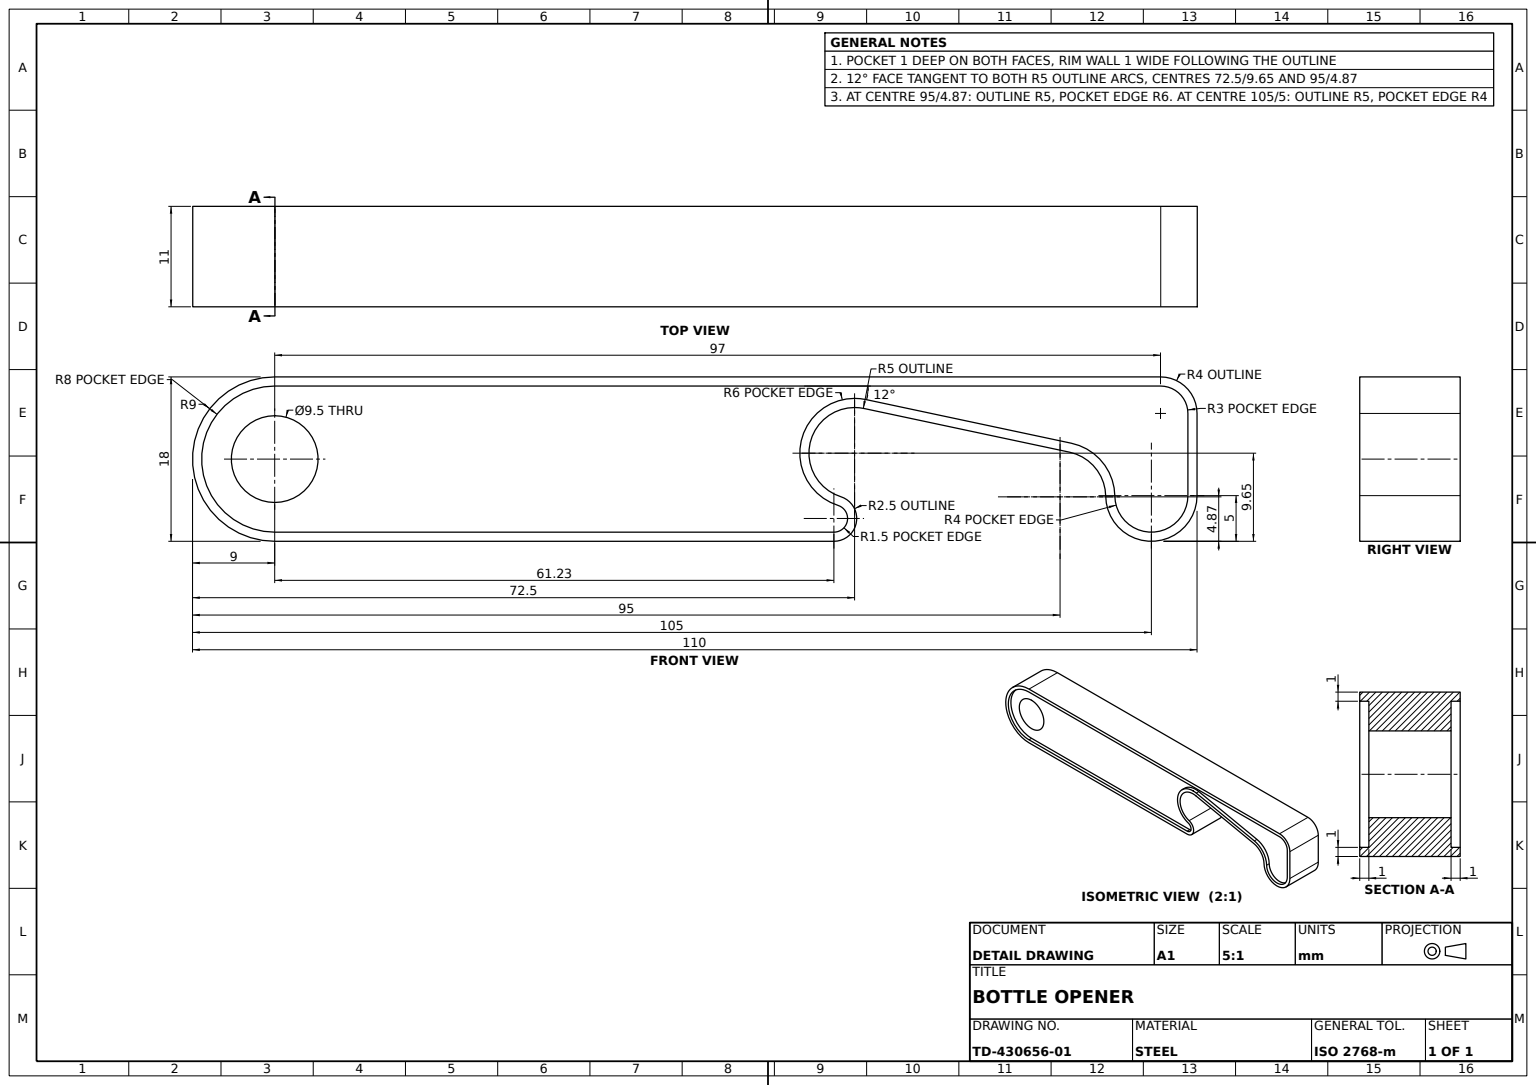
ISO-10303-21;
HEADER;
FILE_DESCRIPTION((''),'2;1');
FILE_NAME('','',(''),(''),'','','');
FILE_SCHEMA(('AUTOMOTIVE_DESIGN'));
ENDSEC;
DATA;
#1=APPLICATION_CONTEXT('');
#2=PRODUCT_CONTEXT('',#1,'mechanical');
#3=PRODUCT('','','',(#2));
#4=PRODUCT_DEFINITION_FORMATION('','',#3);
#5=PRODUCT_DEFINITION_CONTEXT('',#1,'design');
#6=PRODUCT_DEFINITION('','',#4,#5);
#7=PRODUCT_DEFINITION_SHAPE('','',#6);
#8=(LENGTH_UNIT()NAMED_UNIT(*)SI_UNIT(.MILLI.,.METRE.));
#9=(NAMED_UNIT(*)PLANE_ANGLE_UNIT()SI_UNIT($,.RADIAN.));
#10=(NAMED_UNIT(*)SI_UNIT($,.STERADIAN.)SOLID_ANGLE_UNIT());
#11=UNCERTAINTY_MEASURE_WITH_UNIT(LENGTH_MEASURE(1.E-05),#8,'distance_accuracy_value','');
#12=(GEOMETRIC_REPRESENTATION_CONTEXT(3)GLOBAL_UNCERTAINTY_ASSIGNED_CONTEXT((#11))GLOBAL_UNIT_ASSIGNED_CONTEXT((#8,#9,#10))REPRESENTATION_CONTEXT('',''));
#13=CARTESIAN_POINT('',(61.989972,5.5,4.116875));
#14=VERTEX_POINT('',#13);
#15=CARTESIAN_POINT('',(61.989972,-5.5,4.116875));
#16=VERTEX_POINT('',#15);
#17=DIRECTION('',(0.,-1.,0.));
#18=VECTOR('',#17,1000.);
#19=LINE('',#13,#18);
#20=EDGE_CURVE('',#14,#16,#19,.T.);
#21=ORIENTED_EDGE('',*,*,#20,.T.);
#22=CARTESIAN_POINT('',(63.500886,-5.5,-5.649375));
#23=VERTEX_POINT('',#22);
#24=CARTESIAN_POINT('',(63.500886,-5.5,-0.649375));
#25=DIRECTION('',(0.,1.,0.));
#26=DIRECTION('',(0.,0.,1.));
#27=AXIS2_PLACEMENT_3D('',#24,#25,#26);
#28=CIRCLE('',#27,5.);
#29=EDGE_CURVE('',#23,#16,#28,.T.);
#30=ORIENTED_EDGE('',*,*,#29,.F.);
#31=CARTESIAN_POINT('',(63.500886,5.5,-5.649375));
#32=VERTEX_POINT('',#31);
#33=LINE('',#31,#18);
#34=EDGE_CURVE('',#32,#23,#33,.T.);
#35=ORIENTED_EDGE('',*,*,#34,.F.);
#36=CARTESIAN_POINT('',(63.500886,5.5,-0.649375));
#37=AXIS2_PLACEMENT_3D('',#36,#25,#26);
#38=CIRCLE('',#37,5.);
#39=EDGE_CURVE('',#32,#14,#38,.T.);
#40=ORIENTED_EDGE('',*,*,#39,.T.);
#41=EDGE_LOOP('',(#21,#30,#35,#40));
#42=FACE_OUTER_BOUND('',#41,.T.);
#43=DIRECTION('',(0.,0.,-1.));
#44=AXIS2_PLACEMENT_3D('',#36,#17,#43);
#45=CYLINDRICAL_SURFACE('',#44,5.);
#46=ADVANCED_FACE('',(#42),#45,.F.);
#47=CARTESIAN_POINT('',(87.040445,5.5,-0.75759));
#48=VERTEX_POINT('',#47);
#49=CARTESIAN_POINT('',(87.040445,-5.5,-0.75759));
#50=VERTEX_POINT('',#49);
#51=LINE('',#47,#18);
#52=EDGE_CURVE('',#48,#50,#51,.T.);
#53=ORIENTED_EDGE('',*,*,#52,.F.);
#54=CARTESIAN_POINT('',(64.540445,5.5,-5.540113));
#55=VERTEX_POINT('',#54);
#56=CARTESIAN_POINT('',(3.916591,5.5,-18.426111));
#57=DIRECTION('',(0.978147601,0.,0.207911691));
#58=VECTOR('',#57,1000.);
#59=LINE('',#56,#58);
#60=EDGE_CURVE('',#55,#48,#59,.T.);
#61=ORIENTED_EDGE('',*,*,#60,.F.);
#62=CARTESIAN_POINT('',(64.540445,-5.5,-5.540113));
#63=VERTEX_POINT('',#62);
#64=LINE('',#54,#18);
#65=EDGE_CURVE('',#55,#63,#64,.T.);
#66=ORIENTED_EDGE('',*,*,#65,.T.);
#67=CARTESIAN_POINT('',(3.916591,-5.5,-18.426111));
#68=LINE('',#67,#58);
#69=EDGE_CURVE('',#63,#50,#68,.T.);
#70=ORIENTED_EDGE('',*,*,#69,.T.);
#71=EDGE_LOOP('',(#53,#61,#66,#70));
#72=FACE_OUTER_BOUND('',#71,.T.);
#73=DIRECTION('',(0.207911691,0.,-0.978147601));
#74=DIRECTION('',(-0.978147601,0.,-0.207911691));
#75=AXIS2_PLACEMENT_3D('',#56,#73,#74);
#76=PLANE('',#75);
#77=ADVANCED_FACE('',(#72),#76,.F.);
#78=CARTESIAN_POINT('',(64.748357,5.5,-6.51826));
#79=VERTEX_POINT('',#78);
#80=CARTESIAN_POINT('',(63.500886,5.5,-6.649375));
#81=VERTEX_POINT('',#80);
#82=CIRCLE('',#37,6.);
#83=EDGE_CURVE('',#79,#81,#82,.T.);
#84=ORIENTED_EDGE('',*,*,#83,.F.);
#85=CARTESIAN_POINT('',(64.748357,4.5,-6.51826));
#86=VERTEX_POINT('',#85);
#87=LINE('',#78,#18);
#88=EDGE_CURVE('',#79,#86,#87,.T.);
#89=ORIENTED_EDGE('',*,*,#88,.T.);
#90=CARTESIAN_POINT('',(63.500886,4.5,-6.649375));
#91=VERTEX_POINT('',#90);
#92=CARTESIAN_POINT('',(63.500886,4.5,-0.649375));
#93=AXIS2_PLACEMENT_3D('',#92,#25,#26);
#94=CIRCLE('',#93,6.);
#95=EDGE_CURVE('',#86,#91,#94,.T.);
#96=ORIENTED_EDGE('',*,*,#95,.T.);
#97=LINE('',#80,#18);
#98=EDGE_CURVE('',#81,#91,#97,.T.);
#99=ORIENTED_EDGE('',*,*,#98,.F.);
#100=EDGE_LOOP('',(#84,#89,#96,#99));
#101=FACE_OUTER_BOUND('',#100,.T.);
#102=CYLINDRICAL_SURFACE('',#44,6.);
#103=ADVANCED_FACE('',(#101),#102,.T.);
#104=CARTESIAN_POINT('',(100.,-5.5,-5.));
#105=VERTEX_POINT('',#104);
#106=CARTESIAN_POINT('',(97.,-5.5,-8.));
#107=VERTEX_POINT('',#106);
#108=CARTESIAN_POINT('',(97.,-5.5,-5.));
#109=AXIS2_PLACEMENT_3D('',#108,#25,#26);
#110=CIRCLE('',#109,3.);
#111=EDGE_CURVE('',#105,#107,#110,.T.);
#112=ORIENTED_EDGE('',*,*,#111,.F.);
#113=CARTESIAN_POINT('',(100.,-4.5,-5.));
#114=VERTEX_POINT('',#113);
#115=CARTESIAN_POINT('',(100.,5.5,-5.));
#116=LINE('',#115,#18);
#117=EDGE_CURVE('',#114,#105,#116,.T.);
#118=ORIENTED_EDGE('',*,*,#117,.F.);
#119=CARTESIAN_POINT('',(97.,-4.5,-8.));
#120=VERTEX_POINT('',#119);
#121=CARTESIAN_POINT('',(97.,-4.5,-5.));
#122=AXIS2_PLACEMENT_3D('',#121,#25,#26);
#123=CIRCLE('',#122,3.);
#124=EDGE_CURVE('',#114,#120,#123,.T.);
#125=ORIENTED_EDGE('',*,*,#124,.T.);
#126=CARTESIAN_POINT('',(97.,5.5,-8.));
#127=LINE('',#126,#18);
#128=EDGE_CURVE('',#120,#107,#127,.T.);
#129=ORIENTED_EDGE('',*,*,#128,.T.);
#130=EDGE_LOOP('',(#112,#118,#125,#129));
#131=FACE_OUTER_BOUND('',#130,.T.);
#132=CARTESIAN_POINT('',(97.,5.5,-5.));
#133=AXIS2_PLACEMENT_3D('',#132,#17,#43);
#134=CYLINDRICAL_SURFACE('',#133,3.);
#135=ADVANCED_FACE('',(#131),#134,.F.);
#136=CARTESIAN_POINT('',(92.000355,5.5,4.053259));
#137=VERTEX_POINT('',#136);
#138=CARTESIAN_POINT('',(100.,5.5,4.));
#139=VERTEX_POINT('',#138);
#140=CARTESIAN_POINT('',(96.,5.5,4.));
#141=AXIS2_PLACEMENT_3D('',#140,#25,#26);
#142=CIRCLE('',#141,4.);
#143=EDGE_CURVE('',#137,#139,#142,.T.);
#144=ORIENTED_EDGE('',*,*,#143,.T.);
#145=CARTESIAN_POINT('',(100.,4.5,4.));
#146=VERTEX_POINT('',#145);
#147=LINE('',#138,#18);
#148=EDGE_CURVE('',#139,#146,#147,.T.);
#149=ORIENTED_EDGE('',*,*,#148,.T.);
#150=CARTESIAN_POINT('',(92.000355,4.5,4.053259));
#151=VERTEX_POINT('',#150);
#152=CARTESIAN_POINT('',(96.,4.5,4.));
#153=AXIS2_PLACEMENT_3D('',#152,#25,#26);
#154=CIRCLE('',#153,4.);
#155=EDGE_CURVE('',#151,#146,#154,.T.);
#156=ORIENTED_EDGE('',*,*,#155,.F.);
#157=LINE('',#136,#18);
#158=EDGE_CURVE('',#137,#151,#157,.T.);
#159=ORIENTED_EDGE('',*,*,#158,.F.);
#160=EDGE_LOOP('',(#144,#149,#156,#159));
#161=FACE_OUTER_BOUND('',#160,.T.);
#162=AXIS2_PLACEMENT_3D('',#140,#17,#43);
#163=CYLINDRICAL_SURFACE('',#162,4.);
#164=ADVANCED_FACE('',(#161),#163,.F.);
#165=CARTESIAN_POINT('',(0.,5.5,-9.));
#166=VERTEX_POINT('',#165);
#167=CARTESIAN_POINT('',(0.,-5.5,-9.));
#168=VERTEX_POINT('',#167);
#169=LINE('',#165,#18);
#170=EDGE_CURVE('',#166,#168,#169,.T.);
#171=ORIENTED_EDGE('',*,*,#170,.T.);
#172=CARTESIAN_POINT('',(0.,-5.5,9.));
#173=VERTEX_POINT('',#172);
#174=CARTESIAN_POINT('',(0.,-5.5,0.));
#175=AXIS2_PLACEMENT_3D('',#174,#25,#26);
#176=CIRCLE('',#175,9.);
#177=EDGE_CURVE('',#168,#173,#176,.T.);
#178=ORIENTED_EDGE('',*,*,#177,.T.);
#179=CARTESIAN_POINT('',(0.,5.5,9.));
#180=VERTEX_POINT('',#179);
#181=LINE('',#179,#18);
#182=EDGE_CURVE('',#180,#173,#181,.T.);
#183=ORIENTED_EDGE('',*,*,#182,.F.);
#184=CARTESIAN_POINT('',(0.,5.5,0.));
#185=AXIS2_PLACEMENT_3D('',#184,#25,#26);
#186=CIRCLE('',#185,9.);
#187=EDGE_CURVE('',#166,#180,#186,.T.);
#188=ORIENTED_EDGE('',*,*,#187,.F.);
#189=EDGE_LOOP('',(#171,#178,#183,#188));
#190=FACE_OUTER_BOUND('',#189,.T.);
#191=AXIS2_PLACEMENT_3D('',#184,#17,#43);
#192=CYLINDRICAL_SURFACE('',#191,9.);
#193=ADVANCED_FACE('',(#190),#192,.T.);
#194=CARTESIAN_POINT('',(87.248357,-4.5,-1.735738));
#195=VERTEX_POINT('',#194);
#196=CARTESIAN_POINT('',(87.248357,-5.5,-1.735738));
#197=VERTEX_POINT('',#196);
#198=CARTESIAN_POINT('',(87.248357,5.5,-1.735738));
#199=LINE('',#198,#18);
#200=EDGE_CURVE('',#195,#197,#199,.T.);
#201=ORIENTED_EDGE('',*,*,#200,.F.);
#202=CARTESIAN_POINT('',(92.000355,-4.5,4.053259));
#203=VERTEX_POINT('',#202);
#204=CARTESIAN_POINT('',(86.000886,-4.5,4.133148));
#205=AXIS2_PLACEMENT_3D('',#204,#25,#26);
#206=CIRCLE('',#205,6.);
#207=EDGE_CURVE('',#203,#195,#206,.T.);
#208=ORIENTED_EDGE('',*,*,#207,.F.);
#209=CARTESIAN_POINT('',(92.000355,-5.5,4.053259));
#210=VERTEX_POINT('',#209);
#211=EDGE_CURVE('',#203,#210,#157,.T.);
#212=ORIENTED_EDGE('',*,*,#211,.T.);
#213=CARTESIAN_POINT('',(86.000886,-5.5,4.133148));
#214=AXIS2_PLACEMENT_3D('',#213,#25,#26);
#215=CIRCLE('',#214,6.);
#216=EDGE_CURVE('',#210,#197,#215,.T.);
#217=ORIENTED_EDGE('',*,*,#216,.T.);
#218=EDGE_LOOP('',(#201,#208,#212,#217));
#219=FACE_OUTER_BOUND('',#218,.T.);
#220=CARTESIAN_POINT('',(86.000886,5.5,4.133148));
#221=AXIS2_PLACEMENT_3D('',#220,#17,#43);
#222=CYLINDRICAL_SURFACE('',#221,6.);
#223=ADVANCED_FACE('',(#219),#222,.T.);
#224=CARTESIAN_POINT('',(100.,-4.5,4.));
#225=VERTEX_POINT('',#224);
#226=CARTESIAN_POINT('',(100.,-4.5,0.));
#227=VECTOR('',#43,1000.);
#228=LINE('',#226,#227);
#229=EDGE_CURVE('',#225,#114,#228,.T.);
#230=ORIENTED_EDGE('',*,*,#229,.T.);
#231=ORIENTED_EDGE('',*,*,#117,.T.);
#232=CARTESIAN_POINT('',(100.,-5.5,4.));
#233=VERTEX_POINT('',#232);
#234=CARTESIAN_POINT('',(100.,-5.5,0.));
#235=LINE('',#234,#227);
#236=EDGE_CURVE('',#233,#105,#235,.T.);
#237=ORIENTED_EDGE('',*,*,#236,.F.);
#238=EDGE_CURVE('',#225,#233,#147,.T.);
#239=ORIENTED_EDGE('',*,*,#238,.F.);
#240=EDGE_LOOP('',(#230,#231,#237,#239));
#241=FACE_OUTER_BOUND('',#240,.T.);
#242=CARTESIAN_POINT('',(100.,5.5,0.));
#243=DIRECTION('',(-1.,0.,0.));
#244=AXIS2_PLACEMENT_3D('',#242,#243,#26);
#245=PLANE('',#244);
#246=ADVANCED_FACE('',(#241),#245,.T.);
#247=VERTEX_POINT('',#115);
#248=CARTESIAN_POINT('',(100.,4.5,-5.));
#249=VERTEX_POINT('',#248);
#250=EDGE_CURVE('',#247,#249,#116,.T.);
#251=ORIENTED_EDGE('',*,*,#250,.F.);
#252=VERTEX_POINT('',#126);
#253=AXIS2_PLACEMENT_3D('',#132,#25,#26);
#254=CIRCLE('',#253,3.);
#255=EDGE_CURVE('',#247,#252,#254,.T.);
#256=ORIENTED_EDGE('',*,*,#255,.T.);
#257=CARTESIAN_POINT('',(97.,4.5,-8.));
#258=VERTEX_POINT('',#257);
#259=EDGE_CURVE('',#252,#258,#127,.T.);
#260=ORIENTED_EDGE('',*,*,#259,.T.);
#261=CARTESIAN_POINT('',(97.,4.5,-5.));
#262=AXIS2_PLACEMENT_3D('',#261,#25,#26);
#263=CIRCLE('',#262,3.);
#264=EDGE_CURVE('',#249,#258,#263,.T.);
#265=ORIENTED_EDGE('',*,*,#264,.F.);
#266=EDGE_LOOP('',(#251,#256,#260,#265));
#267=FACE_OUTER_BOUND('',#266,.T.);
#268=ADVANCED_FACE('',(#267),#134,.F.);
#269=CARTESIAN_POINT('',(87.248357,4.5,-1.735738));
#270=VERTEX_POINT('',#269);
#271=CARTESIAN_POINT('',(86.000886,4.5,4.133148));
#272=AXIS2_PLACEMENT_3D('',#271,#25,#26);
#273=CIRCLE('',#272,6.);
#274=EDGE_CURVE('',#151,#270,#273,.T.);
#275=ORIENTED_EDGE('',*,*,#274,.T.);
#276=VERTEX_POINT('',#198);
#277=EDGE_CURVE('',#276,#270,#199,.T.);
#278=ORIENTED_EDGE('',*,*,#277,.F.);
#279=AXIS2_PLACEMENT_3D('',#220,#25,#26);
#280=CIRCLE('',#279,6.);
#281=EDGE_CURVE('',#137,#276,#280,.T.);
#282=ORIENTED_EDGE('',*,*,#281,.F.);
#283=ORIENTED_EDGE('',*,*,#158,.T.);
#284=EDGE_LOOP('',(#275,#278,#282,#283));
#285=FACE_OUTER_BOUND('',#284,.T.);
#286=ADVANCED_FACE('',(#285),#222,.T.);
#287=CARTESIAN_POINT('',(61.234514,-5.5,9.));
#288=VERTEX_POINT('',#287);
#289=CARTESIAN_POINT('',(61.234514,-5.5,6.5));
#290=AXIS2_PLACEMENT_3D('',#289,#25,#26);
#291=CIRCLE('',#290,2.5);
#292=EDGE_CURVE('',#288,#16,#291,.T.);
#293=ORIENTED_EDGE('',*,*,#292,.T.);
#294=ORIENTED_EDGE('',*,*,#20,.F.);
#295=CARTESIAN_POINT('',(61.234514,5.5,9.));
#296=VERTEX_POINT('',#295);
#297=CARTESIAN_POINT('',(61.234514,5.5,6.5));
#298=AXIS2_PLACEMENT_3D('',#297,#25,#26);
#299=CIRCLE('',#298,2.5);
#300=EDGE_CURVE('',#296,#14,#299,.T.);
#301=ORIENTED_EDGE('',*,*,#300,.F.);
#302=LINE('',#295,#18);
#303=EDGE_CURVE('',#296,#288,#302,.T.);
#304=ORIENTED_EDGE('',*,*,#303,.T.);
#305=EDGE_LOOP('',(#293,#294,#301,#304));
#306=FACE_OUTER_BOUND('',#305,.T.);
#307=AXIS2_PLACEMENT_3D('',#297,#17,#43);
#308=CYLINDRICAL_SURFACE('',#307,2.5);
#309=ADVANCED_FACE('',(#306),#308,.T.);
#310=CARTESIAN_POINT('',(0.,4.5,4.75));
#311=VERTEX_POINT('',#310);
#312=CARTESIAN_POINT('',(0.,4.5,-4.75));
#313=VERTEX_POINT('',#312);
#314=CARTESIAN_POINT('',(0.,4.5,0.));
#315=AXIS2_PLACEMENT_3D('',#314,#25,#26);
#316=CIRCLE('',#315,4.75);
#317=EDGE_CURVE('',#311,#313,#316,.T.);
#318=ORIENTED_EDGE('',*,*,#317,.F.);
#319=EDGE_CURVE('',#313,#311,#316,.T.);
#320=ORIENTED_EDGE('',*,*,#319,.F.);
#321=EDGE_LOOP('',(#318,#320));
#322=FACE_BOUND('',#321,.T.);
#323=CARTESIAN_POINT('',(0.,4.5,-8.));
#324=VERTEX_POINT('',#323);
#325=DIRECTION('',(1.,0.,0.));
#326=VECTOR('',#325,1000.);
#327=LINE('',#323,#326);
#328=EDGE_CURVE('',#324,#258,#327,.T.);
#329=ORIENTED_EDGE('',*,*,#328,.F.);
#330=CARTESIAN_POINT('',(0.,4.5,8.));
#331=VERTEX_POINT('',#330);
#332=CIRCLE('',#315,8.);
#333=EDGE_CURVE('',#324,#331,#332,.T.);
#334=ORIENTED_EDGE('',*,*,#333,.T.);
#335=CARTESIAN_POINT('',(61.234514,4.5,8.));
#336=VERTEX_POINT('',#335);
#337=LINE('',#330,#326);
#338=EDGE_CURVE('',#331,#336,#337,.T.);
#339=ORIENTED_EDGE('',*,*,#338,.T.);
#340=CARTESIAN_POINT('',(61.687789,4.5,5.070125));
#341=VERTEX_POINT('',#340);
#342=CARTESIAN_POINT('',(61.234514,4.5,6.5));
#343=AXIS2_PLACEMENT_3D('',#342,#25,#26);
#344=CIRCLE('',#343,1.5);
#345=EDGE_CURVE('',#336,#341,#344,.T.);
#346=ORIENTED_EDGE('',*,*,#345,.T.);
#347=EDGE_CURVE('',#91,#341,#94,.T.);
#348=ORIENTED_EDGE('',*,*,#347,.F.);
#349=ORIENTED_EDGE('',*,*,#95,.F.);
#350=CARTESIAN_POINT('',(4.124502,4.5,-19.404258));
#351=LINE('',#350,#58);
#352=EDGE_CURVE('',#86,#270,#351,.T.);
#353=ORIENTED_EDGE('',*,*,#352,.T.);
#354=ORIENTED_EDGE('',*,*,#274,.F.);
#355=ORIENTED_EDGE('',*,*,#155,.T.);
#356=CARTESIAN_POINT('',(100.,4.5,0.));
#357=LINE('',#356,#227);
#358=EDGE_CURVE('',#146,#249,#357,.T.);
#359=ORIENTED_EDGE('',*,*,#358,.T.);
#360=ORIENTED_EDGE('',*,*,#264,.T.);
#361=EDGE_LOOP('',(#329,#334,#339,#346,#348,#349,#353,#354,#355,#359,#360));
#362=FACE_OUTER_BOUND('',#361,.T.);
#363=PLANE('',#315);
#364=ADVANCED_FACE('',(#322,#362),#363,.T.);
#365=ORIENTED_EDGE('',*,*,#317,.T.);
#366=CARTESIAN_POINT('',(0.,-4.5,-4.75));
#367=VERTEX_POINT('',#366);
#368=LINE('',#312,#18);
#369=EDGE_CURVE('',#313,#367,#368,.T.);
#370=ORIENTED_EDGE('',*,*,#369,.T.);
#371=CARTESIAN_POINT('',(0.,-4.5,4.75));
#372=VERTEX_POINT('',#371);
#373=CARTESIAN_POINT('',(0.,-4.5,0.));
#374=AXIS2_PLACEMENT_3D('',#373,#25,#26);
#375=CIRCLE('',#374,4.75);
#376=EDGE_CURVE('',#372,#367,#375,.T.);
#377=ORIENTED_EDGE('',*,*,#376,.F.);
#378=LINE('',#310,#18);
#379=EDGE_CURVE('',#311,#372,#378,.T.);
#380=ORIENTED_EDGE('',*,*,#379,.F.);
#381=EDGE_LOOP('',(#365,#370,#377,#380));
#382=FACE_OUTER_BOUND('',#381,.T.);
#383=AXIS2_PLACEMENT_3D('',#314,#17,#43);
#384=CYLINDRICAL_SURFACE('',#383,4.75);
#385=ADVANCED_FACE('',(#382),#384,.F.);
#386=ORIENTED_EDGE('',*,*,#281,.T.);
#387=CARTESIAN_POINT('',(4.124502,5.5,-19.404258));
#388=LINE('',#387,#58);
#389=EDGE_CURVE('',#79,#276,#388,.T.);
#390=ORIENTED_EDGE('',*,*,#389,.F.);
#391=ORIENTED_EDGE('',*,*,#83,.T.);
#392=CARTESIAN_POINT('',(61.687789,5.5,5.070125));
#393=VERTEX_POINT('',#392);
#394=EDGE_CURVE('',#81,#393,#82,.T.);
#395=ORIENTED_EDGE('',*,*,#394,.T.);
#396=CARTESIAN_POINT('',(61.234514,5.5,8.));
#397=VERTEX_POINT('',#396);
#398=CIRCLE('',#298,1.5);
#399=EDGE_CURVE('',#397,#393,#398,.T.);
#400=ORIENTED_EDGE('',*,*,#399,.F.);
#401=CARTESIAN_POINT('',(0.,5.5,8.));
#402=VERTEX_POINT('',#401);
#403=LINE('',#401,#326);
#404=EDGE_CURVE('',#402,#397,#403,.T.);
#405=ORIENTED_EDGE('',*,*,#404,.F.);
#406=CARTESIAN_POINT('',(0.,5.5,-8.));
#407=VERTEX_POINT('',#406);
#408=CIRCLE('',#185,8.);
#409=EDGE_CURVE('',#407,#402,#408,.T.);
#410=ORIENTED_EDGE('',*,*,#409,.F.);
#411=LINE('',#406,#326);
#412=EDGE_CURVE('',#407,#252,#411,.T.);
#413=ORIENTED_EDGE('',*,*,#412,.T.);
#414=ORIENTED_EDGE('',*,*,#255,.F.);
#415=LINE('',#242,#227);
#416=EDGE_CURVE('',#139,#247,#415,.T.);
#417=ORIENTED_EDGE('',*,*,#416,.F.);
#418=ORIENTED_EDGE('',*,*,#143,.F.);
#419=EDGE_LOOP('',(#386,#390,#391,#395,#400,#405,#410,#413,#414,#417,#418));
#420=FACE_BOUND('',#419,.T.);
#421=ORIENTED_EDGE('',*,*,#60,.T.);
#422=CARTESIAN_POINT('',(91.000443,5.5,4.066574));
#423=VERTEX_POINT('',#422);
#424=CIRCLE('',#279,5.);
#425=EDGE_CURVE('',#423,#48,#424,.T.);
#426=ORIENTED_EDGE('',*,*,#425,.F.);
#427=CARTESIAN_POINT('',(101.,5.5,4.));
#428=VERTEX_POINT('',#427);
#429=CIRCLE('',#141,5.);
#430=EDGE_CURVE('',#423,#428,#429,.T.);
#431=ORIENTED_EDGE('',*,*,#430,.T.);
#432=CARTESIAN_POINT('',(101.,5.5,-5.));
#433=VERTEX_POINT('',#432);
#434=CARTESIAN_POINT('',(101.,5.5,0.));
#435=LINE('',#434,#227);
#436=EDGE_CURVE('',#428,#433,#435,.T.);
#437=ORIENTED_EDGE('',*,*,#436,.T.);
#438=CARTESIAN_POINT('',(97.,5.5,-9.));
#439=VERTEX_POINT('',#438);
#440=CIRCLE('',#253,4.);
#441=EDGE_CURVE('',#433,#439,#440,.T.);
#442=ORIENTED_EDGE('',*,*,#441,.T.);
#443=LINE('',#165,#326);
#444=EDGE_CURVE('',#166,#439,#443,.T.);
#445=ORIENTED_EDGE('',*,*,#444,.F.);
#446=ORIENTED_EDGE('',*,*,#187,.T.);
#447=LINE('',#179,#326);
#448=EDGE_CURVE('',#180,#296,#447,.T.);
#449=ORIENTED_EDGE('',*,*,#448,.T.);
#450=ORIENTED_EDGE('',*,*,#300,.T.);
#451=ORIENTED_EDGE('',*,*,#39,.F.);
#452=EDGE_CURVE('',#55,#32,#38,.T.);
#453=ORIENTED_EDGE('',*,*,#452,.F.);
#454=EDGE_LOOP('',(#421,#426,#431,#437,#442,#445,#446,#449,#450,#451,#453));
#455=FACE_OUTER_BOUND('',#454,.T.);
#456=PLANE('',#185);
#457=ADVANCED_FACE('',(#420,#455),#456,.T.);
#458=ORIENTED_EDGE('',*,*,#170,.F.);
#459=ORIENTED_EDGE('',*,*,#444,.T.);
#460=CARTESIAN_POINT('',(97.,-5.5,-9.));
#461=VERTEX_POINT('',#460);
#462=LINE('',#438,#18);
#463=EDGE_CURVE('',#439,#461,#462,.T.);
#464=ORIENTED_EDGE('',*,*,#463,.T.);
#465=LINE('',#167,#326);
#466=EDGE_CURVE('',#168,#461,#465,.T.);
#467=ORIENTED_EDGE('',*,*,#466,.F.);
#468=EDGE_LOOP('',(#458,#459,#464,#467));
#469=FACE_OUTER_BOUND('',#468,.T.);
#470=AXIS2_PLACEMENT_3D('',#165,#43,#243);
#471=PLANE('',#470);
#472=ADVANCED_FACE('',(#469),#471,.T.);
#473=CARTESIAN_POINT('',(63.500886,-4.5,-6.649375));
#474=VERTEX_POINT('',#473);
#475=CARTESIAN_POINT('',(63.500886,-5.5,-6.649375));
#476=VERTEX_POINT('',#475);
#477=EDGE_CURVE('',#474,#476,#97,.T.);
#478=ORIENTED_EDGE('',*,*,#477,.F.);
#479=CARTESIAN_POINT('',(64.748357,-4.5,-6.51826));
#480=VERTEX_POINT('',#479);
#481=CARTESIAN_POINT('',(63.500886,-4.5,-0.649375));
#482=AXIS2_PLACEMENT_3D('',#481,#25,#26);
#483=CIRCLE('',#482,6.);
#484=EDGE_CURVE('',#480,#474,#483,.T.);
#485=ORIENTED_EDGE('',*,*,#484,.F.);
#486=CARTESIAN_POINT('',(64.748357,-5.5,-6.51826));
#487=VERTEX_POINT('',#486);
#488=EDGE_CURVE('',#480,#487,#87,.T.);
#489=ORIENTED_EDGE('',*,*,#488,.T.);
#490=CIRCLE('',#27,6.);
#491=EDGE_CURVE('',#487,#476,#490,.T.);
#492=ORIENTED_EDGE('',*,*,#491,.T.);
#493=EDGE_LOOP('',(#478,#485,#489,#492));
#494=FACE_OUTER_BOUND('',#493,.T.);
#495=ADVANCED_FACE('',(#494),#102,.T.);
#496=ORIENTED_EDGE('',*,*,#98,.T.);
#497=ORIENTED_EDGE('',*,*,#347,.T.);
#498=LINE('',#392,#18);
#499=EDGE_CURVE('',#393,#341,#498,.T.);
#500=ORIENTED_EDGE('',*,*,#499,.F.);
#501=ORIENTED_EDGE('',*,*,#394,.F.);
#502=EDGE_LOOP('',(#496,#497,#500,#501));
#503=FACE_OUTER_BOUND('',#502,.T.);
#504=ADVANCED_FACE('',(#503),#102,.T.);
#505=ORIENTED_EDGE('',*,*,#207,.T.);
#506=CARTESIAN_POINT('',(4.124502,-4.5,-19.404258));
#507=LINE('',#506,#58);
#508=EDGE_CURVE('',#480,#195,#507,.T.);
#509=ORIENTED_EDGE('',*,*,#508,.F.);
#510=ORIENTED_EDGE('',*,*,#484,.T.);
#511=CARTESIAN_POINT('',(61.687789,-4.5,5.070125));
#512=VERTEX_POINT('',#511);
#513=EDGE_CURVE('',#474,#512,#483,.T.);
#514=ORIENTED_EDGE('',*,*,#513,.T.);
#515=CARTESIAN_POINT('',(61.234514,-4.5,8.));
#516=VERTEX_POINT('',#515);
#517=CARTESIAN_POINT('',(61.234514,-4.5,6.5));
#518=AXIS2_PLACEMENT_3D('',#517,#25,#26);
#519=CIRCLE('',#518,1.5);
#520=EDGE_CURVE('',#516,#512,#519,.T.);
#521=ORIENTED_EDGE('',*,*,#520,.F.);
#522=CARTESIAN_POINT('',(0.,-4.5,8.));
#523=VERTEX_POINT('',#522);
#524=LINE('',#522,#326);
#525=EDGE_CURVE('',#523,#516,#524,.T.);
#526=ORIENTED_EDGE('',*,*,#525,.F.);
#527=CARTESIAN_POINT('',(0.,-4.5,-8.));
#528=VERTEX_POINT('',#527);
#529=CIRCLE('',#374,8.);
#530=EDGE_CURVE('',#528,#523,#529,.T.);
#531=ORIENTED_EDGE('',*,*,#530,.F.);
#532=LINE('',#527,#326);
#533=EDGE_CURVE('',#528,#120,#532,.T.);
#534=ORIENTED_EDGE('',*,*,#533,.T.);
#535=ORIENTED_EDGE('',*,*,#124,.F.);
#536=ORIENTED_EDGE('',*,*,#229,.F.);
#537=CARTESIAN_POINT('',(96.,-4.5,4.));
#538=AXIS2_PLACEMENT_3D('',#537,#25,#26);
#539=CIRCLE('',#538,4.);
#540=EDGE_CURVE('',#203,#225,#539,.T.);
#541=ORIENTED_EDGE('',*,*,#540,.F.);
#542=EDGE_LOOP('',(#505,#509,#510,#514,#521,#526,#531,#534,#535,#536,#541));
#543=FACE_OUTER_BOUND('',#542,.T.);
#544=ORIENTED_EDGE('',*,*,#376,.T.);
#545=EDGE_CURVE('',#367,#372,#375,.T.);
#546=ORIENTED_EDGE('',*,*,#545,.T.);
#547=EDGE_LOOP('',(#544,#546));
#548=FACE_BOUND('',#547,.T.);
#549=PLANE('',#374);
#550=ADVANCED_FACE('',(#543,#548),#549,.F.);
#551=ORIENTED_EDGE('',*,*,#277,.T.);
#552=ORIENTED_EDGE('',*,*,#352,.F.);
#553=ORIENTED_EDGE('',*,*,#88,.F.);
#554=ORIENTED_EDGE('',*,*,#389,.T.);
#555=EDGE_LOOP('',(#551,#552,#553,#554));
#556=FACE_OUTER_BOUND('',#555,.T.);
#557=AXIS2_PLACEMENT_3D('',#387,#73,#74);
#558=PLANE('',#557);
#559=ADVANCED_FACE('',(#556),#558,.T.);
#560=ORIENTED_EDGE('',*,*,#177,.F.);
#561=ORIENTED_EDGE('',*,*,#466,.T.);
#562=CARTESIAN_POINT('',(101.,-5.5,-5.));
#563=VERTEX_POINT('',#562);
#564=CIRCLE('',#109,4.);
#565=EDGE_CURVE('',#563,#461,#564,.T.);
#566=ORIENTED_EDGE('',*,*,#565,.F.);
#567=CARTESIAN_POINT('',(101.,-5.5,4.));
#568=VERTEX_POINT('',#567);
#569=CARTESIAN_POINT('',(101.,-5.5,0.));
#570=LINE('',#569,#227);
#571=EDGE_CURVE('',#568,#563,#570,.T.);
#572=ORIENTED_EDGE('',*,*,#571,.F.);
#573=CARTESIAN_POINT('',(91.000443,-5.5,4.066574));
#574=VERTEX_POINT('',#573);
#575=CARTESIAN_POINT('',(96.,-5.5,4.));
#576=AXIS2_PLACEMENT_3D('',#575,#25,#26);
#577=CIRCLE('',#576,5.);
#578=EDGE_CURVE('',#574,#568,#577,.T.);
#579=ORIENTED_EDGE('',*,*,#578,.F.);
#580=CIRCLE('',#214,5.);
#581=EDGE_CURVE('',#574,#50,#580,.T.);
#582=ORIENTED_EDGE('',*,*,#581,.T.);
#583=ORIENTED_EDGE('',*,*,#69,.F.);
#584=EDGE_CURVE('',#63,#23,#28,.T.);
#585=ORIENTED_EDGE('',*,*,#584,.T.);
#586=ORIENTED_EDGE('',*,*,#29,.T.);
#587=ORIENTED_EDGE('',*,*,#292,.F.);
#588=LINE('',#172,#326);
#589=EDGE_CURVE('',#173,#288,#588,.T.);
#590=ORIENTED_EDGE('',*,*,#589,.F.);
#591=EDGE_LOOP('',(#560,#561,#566,#572,#579,#582,#583,#585,#586,#587,#590));
#592=FACE_OUTER_BOUND('',#591,.T.);
#593=CARTESIAN_POINT('',(4.124502,-5.5,-19.404258));
#594=LINE('',#593,#58);
#595=EDGE_CURVE('',#487,#197,#594,.T.);
#596=ORIENTED_EDGE('',*,*,#595,.T.);
#597=ORIENTED_EDGE('',*,*,#216,.F.);
#598=CIRCLE('',#576,4.);
#599=EDGE_CURVE('',#210,#233,#598,.T.);
#600=ORIENTED_EDGE('',*,*,#599,.T.);
#601=ORIENTED_EDGE('',*,*,#236,.T.);
#602=ORIENTED_EDGE('',*,*,#111,.T.);
#603=CARTESIAN_POINT('',(0.,-5.5,-8.));
#604=VERTEX_POINT('',#603);
#605=LINE('',#603,#326);
#606=EDGE_CURVE('',#604,#107,#605,.T.);
#607=ORIENTED_EDGE('',*,*,#606,.F.);
#608=CARTESIAN_POINT('',(0.,-5.5,8.));
#609=VERTEX_POINT('',#608);
#610=CIRCLE('',#175,8.);
#611=EDGE_CURVE('',#604,#609,#610,.T.);
#612=ORIENTED_EDGE('',*,*,#611,.T.);
#613=CARTESIAN_POINT('',(61.234514,-5.5,8.));
#614=VERTEX_POINT('',#613);
#615=LINE('',#608,#326);
#616=EDGE_CURVE('',#609,#614,#615,.T.);
#617=ORIENTED_EDGE('',*,*,#616,.T.);
#618=CARTESIAN_POINT('',(61.687789,-5.5,5.070125));
#619=VERTEX_POINT('',#618);
#620=CIRCLE('',#290,1.5);
#621=EDGE_CURVE('',#614,#619,#620,.T.);
#622=ORIENTED_EDGE('',*,*,#621,.T.);
#623=EDGE_CURVE('',#476,#619,#490,.T.);
#624=ORIENTED_EDGE('',*,*,#623,.F.);
#625=ORIENTED_EDGE('',*,*,#491,.F.);
#626=EDGE_LOOP('',(#596,#597,#600,#601,#602,#607,#612,#617,#622,#624,#625));
#627=FACE_BOUND('',#626,.T.);
#628=PLANE('',#175);
#629=ADVANCED_FACE('',(#592,#627),#628,.F.);
#630=LINE('',#396,#18);
#631=EDGE_CURVE('',#397,#336,#630,.T.);
#632=ORIENTED_EDGE('',*,*,#631,.T.);
#633=ORIENTED_EDGE('',*,*,#338,.F.);
#634=LINE('',#401,#18);
#635=EDGE_CURVE('',#402,#331,#634,.T.);
#636=ORIENTED_EDGE('',*,*,#635,.F.);
#637=ORIENTED_EDGE('',*,*,#404,.T.);
#638=EDGE_LOOP('',(#632,#633,#636,#637));
#639=FACE_OUTER_BOUND('',#638,.T.);
#640=AXIS2_PLACEMENT_3D('',#401,#43,#243);
#641=PLANE('',#640);
#642=ADVANCED_FACE('',(#639),#641,.T.);
#643=ORIENTED_EDGE('',*,*,#441,.F.);
#644=LINE('',#432,#18);
#645=EDGE_CURVE('',#433,#563,#644,.T.);
#646=ORIENTED_EDGE('',*,*,#645,.T.);
#647=ORIENTED_EDGE('',*,*,#565,.T.);
#648=ORIENTED_EDGE('',*,*,#463,.F.);
#649=EDGE_LOOP('',(#643,#646,#647,#648));
#650=FACE_OUTER_BOUND('',#649,.T.);
#651=CYLINDRICAL_SURFACE('',#133,4.);
#652=ADVANCED_FACE('',(#650),#651,.T.);
#653=ORIENTED_EDGE('',*,*,#259,.F.);
#654=ORIENTED_EDGE('',*,*,#412,.F.);
#655=LINE('',#406,#18);
#656=EDGE_CURVE('',#407,#324,#655,.T.);
#657=ORIENTED_EDGE('',*,*,#656,.T.);
#658=ORIENTED_EDGE('',*,*,#328,.T.);
#659=EDGE_LOOP('',(#653,#654,#657,#658));
#660=FACE_OUTER_BOUND('',#659,.T.);
#661=AXIS2_PLACEMENT_3D('',#406,#43,#243);
#662=PLANE('',#661);
#663=ADVANCED_FACE('',(#660),#662,.F.);
#664=ORIENTED_EDGE('',*,*,#513,.F.);
#665=ORIENTED_EDGE('',*,*,#477,.T.);
#666=ORIENTED_EDGE('',*,*,#623,.T.);
#667=EDGE_CURVE('',#512,#619,#498,.T.);
#668=ORIENTED_EDGE('',*,*,#667,.F.);
#669=EDGE_LOOP('',(#664,#665,#666,#668));
#670=FACE_OUTER_BOUND('',#669,.T.);
#671=ADVANCED_FACE('',(#670),#102,.T.);
#672=LINE('',#427,#18);
#673=EDGE_CURVE('',#428,#568,#672,.T.);
#674=ORIENTED_EDGE('',*,*,#673,.F.);
#675=ORIENTED_EDGE('',*,*,#430,.F.);
#676=LINE('',#422,#18);
#677=EDGE_CURVE('',#423,#574,#676,.T.);
#678=ORIENTED_EDGE('',*,*,#677,.T.);
#679=ORIENTED_EDGE('',*,*,#578,.T.);
#680=EDGE_LOOP('',(#674,#675,#678,#679));
#681=FACE_OUTER_BOUND('',#680,.T.);
#682=CYLINDRICAL_SURFACE('',#162,5.);
#683=ADVANCED_FACE('',(#681),#682,.T.);
#684=ORIENTED_EDGE('',*,*,#448,.F.);
#685=ORIENTED_EDGE('',*,*,#182,.T.);
#686=ORIENTED_EDGE('',*,*,#589,.T.);
#687=ORIENTED_EDGE('',*,*,#303,.F.);
#688=EDGE_LOOP('',(#684,#685,#686,#687));
#689=FACE_OUTER_BOUND('',#688,.T.);
#690=AXIS2_PLACEMENT_3D('',#179,#43,#243);
#691=PLANE('',#690);
#692=ADVANCED_FACE('',(#689),#691,.F.);
#693=ORIENTED_EDGE('',*,*,#238,.T.);
#694=ORIENTED_EDGE('',*,*,#599,.F.);
#695=ORIENTED_EDGE('',*,*,#211,.F.);
#696=ORIENTED_EDGE('',*,*,#540,.T.);
#697=EDGE_LOOP('',(#693,#694,#695,#696));
#698=FACE_OUTER_BOUND('',#697,.T.);
#699=ADVANCED_FACE('',(#698),#163,.F.);
#700=ORIENTED_EDGE('',*,*,#673,.T.);
#701=ORIENTED_EDGE('',*,*,#571,.T.);
#702=ORIENTED_EDGE('',*,*,#645,.F.);
#703=ORIENTED_EDGE('',*,*,#436,.F.);
#704=EDGE_LOOP('',(#700,#701,#702,#703));
#705=FACE_OUTER_BOUND('',#704,.T.);
#706=AXIS2_PLACEMENT_3D('',#434,#243,#26);
#707=PLANE('',#706);
#708=ADVANCED_FACE('',(#705),#707,.F.);
#709=EDGE_CURVE('',#523,#609,#634,.T.);
#710=ORIENTED_EDGE('',*,*,#709,.T.);
#711=ORIENTED_EDGE('',*,*,#611,.F.);
#712=EDGE_CURVE('',#528,#604,#655,.T.);
#713=ORIENTED_EDGE('',*,*,#712,.F.);
#714=ORIENTED_EDGE('',*,*,#530,.T.);
#715=EDGE_LOOP('',(#710,#711,#713,#714));
#716=FACE_OUTER_BOUND('',#715,.T.);
#717=CYLINDRICAL_SURFACE('',#191,8.);
#718=ADVANCED_FACE('',(#716),#717,.F.);
#719=ORIENTED_EDGE('',*,*,#635,.T.);
#720=ORIENTED_EDGE('',*,*,#333,.F.);
#721=ORIENTED_EDGE('',*,*,#656,.F.);
#722=ORIENTED_EDGE('',*,*,#409,.T.);
#723=EDGE_LOOP('',(#719,#720,#721,#722));
#724=FACE_OUTER_BOUND('',#723,.T.);
#725=ADVANCED_FACE('',(#724),#717,.F.);
#726=ORIENTED_EDGE('',*,*,#425,.T.);
#727=ORIENTED_EDGE('',*,*,#52,.T.);
#728=ORIENTED_EDGE('',*,*,#581,.F.);
#729=ORIENTED_EDGE('',*,*,#677,.F.);
#730=EDGE_LOOP('',(#726,#727,#728,#729));
#731=FACE_OUTER_BOUND('',#730,.T.);
#732=CYLINDRICAL_SURFACE('',#221,5.);
#733=ADVANCED_FACE('',(#731),#732,.F.);
#734=ORIENTED_EDGE('',*,*,#452,.T.);
#735=ORIENTED_EDGE('',*,*,#34,.T.);
#736=ORIENTED_EDGE('',*,*,#584,.F.);
#737=ORIENTED_EDGE('',*,*,#65,.F.);
#738=EDGE_LOOP('',(#734,#735,#736,#737));
#739=FACE_OUTER_BOUND('',#738,.T.);
#740=ADVANCED_FACE('',(#739),#45,.F.);
#741=ORIENTED_EDGE('',*,*,#606,.T.);
#742=ORIENTED_EDGE('',*,*,#128,.F.);
#743=ORIENTED_EDGE('',*,*,#533,.F.);
#744=ORIENTED_EDGE('',*,*,#712,.T.);
#745=EDGE_LOOP('',(#741,#742,#743,#744));
#746=FACE_OUTER_BOUND('',#745,.T.);
#747=ADVANCED_FACE('',(#746),#662,.F.);
#748=ORIENTED_EDGE('',*,*,#250,.T.);
#749=ORIENTED_EDGE('',*,*,#358,.F.);
#750=ORIENTED_EDGE('',*,*,#148,.F.);
#751=ORIENTED_EDGE('',*,*,#416,.T.);
#752=EDGE_LOOP('',(#748,#749,#750,#751));
#753=FACE_OUTER_BOUND('',#752,.T.);
#754=ADVANCED_FACE('',(#753),#245,.T.);
#755=ORIENTED_EDGE('',*,*,#379,.T.);
#756=ORIENTED_EDGE('',*,*,#545,.F.);
#757=ORIENTED_EDGE('',*,*,#369,.F.);
#758=ORIENTED_EDGE('',*,*,#319,.T.);
#759=EDGE_LOOP('',(#755,#756,#757,#758));
#760=FACE_OUTER_BOUND('',#759,.T.);
#761=ADVANCED_FACE('',(#760),#384,.F.);
#762=ORIENTED_EDGE('',*,*,#200,.T.);
#763=ORIENTED_EDGE('',*,*,#595,.F.);
#764=ORIENTED_EDGE('',*,*,#488,.F.);
#765=ORIENTED_EDGE('',*,*,#508,.T.);
#766=EDGE_LOOP('',(#762,#763,#764,#765));
#767=FACE_OUTER_BOUND('',#766,.T.);
#768=ADVANCED_FACE('',(#767),#558,.T.);
#769=ORIENTED_EDGE('',*,*,#399,.T.);
#770=ORIENTED_EDGE('',*,*,#499,.T.);
#771=ORIENTED_EDGE('',*,*,#345,.F.);
#772=ORIENTED_EDGE('',*,*,#631,.F.);
#773=EDGE_LOOP('',(#769,#770,#771,#772));
#774=FACE_OUTER_BOUND('',#773,.T.);
#775=CYLINDRICAL_SURFACE('',#307,1.5);
#776=ADVANCED_FACE('',(#774),#775,.F.);
#777=ORIENTED_EDGE('',*,*,#667,.T.);
#778=ORIENTED_EDGE('',*,*,#621,.F.);
#779=EDGE_CURVE('',#516,#614,#630,.T.);
#780=ORIENTED_EDGE('',*,*,#779,.F.);
#781=ORIENTED_EDGE('',*,*,#520,.T.);
#782=EDGE_LOOP('',(#777,#778,#780,#781));
#783=FACE_OUTER_BOUND('',#782,.T.);
#784=ADVANCED_FACE('',(#783),#775,.F.);
#785=ORIENTED_EDGE('',*,*,#709,.F.);
#786=ORIENTED_EDGE('',*,*,#525,.T.);
#787=ORIENTED_EDGE('',*,*,#779,.T.);
#788=ORIENTED_EDGE('',*,*,#616,.F.);
#789=EDGE_LOOP('',(#785,#786,#787,#788));
#790=FACE_OUTER_BOUND('',#789,.T.);
#791=ADVANCED_FACE('',(#790),#641,.T.);
#792=CLOSED_SHELL('',(#46,#77,#103,#135,#164,#193,#223,#246,#268,#286,#309,#364,#385,#457,#472,#495,#504,#550,#559,#629,#642,#652,#663,#671,#683,#692,#699,#708,#718,#725,#733,#740,#747,#754,#761,#768,#776,#784,#791));
#793=MANIFOLD_SOLID_BREP('',#792);
#794=ADVANCED_BREP_SHAPE_REPRESENTATION('',(#793),#12);
#795=SHAPE_DEFINITION_REPRESENTATION(#7,#794);
ENDSEC;
END-ISO-10303-21;
